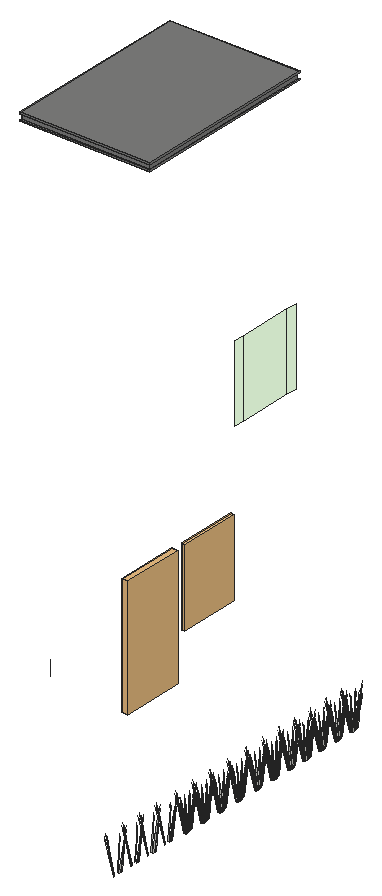
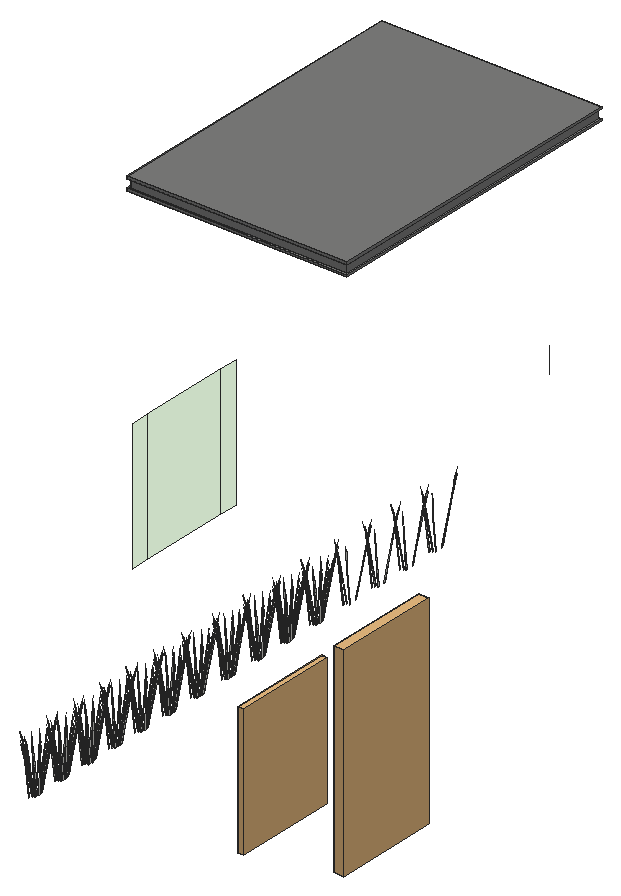
# SketchUp Ruby script. Lengths in inches.
U = 1.inch
M = Sketchup.active_model
def pt(a) = Geom::Point3d.new(a.map { |v| v * U })
def face(e, loops, mat)
  f = e.add_face(loops[0].map { |a| pt(a) })
  loops[1..].each { |l| e.add_face(l.map { |a| pt(a) }).erase! }
  f.material = f.back_material = mat if mat
  f
end
# faces: each face lists its corners as indices into pts; further lists are holes
def faces(e, pts, list, mat = nil) = list.each { |f| face(e, (f[0].is_a?(Array) ? f : [f]).map { |l| l.map { |i| pts[i] } }, mat) }
# xy, xz, yz: faces in a plane at the given z, y or x. An outline is a flat list of corners, or four numbers for a rectangle; further outlines are holes
def ring(l) = l.size == 4 ? [[l[0], l[1]], [l[2], l[1]], [l[2], l[3]], [l[0], l[3]]] : l.each_slice(2).to_a
def flat(e, list, mat, &to3) = list.each { |f| face(e, (f[0].is_a?(Array) ? f : [f]).map { |l| ring(l).map { |u, v| to3.(u, v) } }, mat) }
def xy(e, z, list, mat = nil) = flat(e, list, mat) { |x, y| [x, y, z] }
def xz(e, y, list, mat = nil) = flat(e, list, mat) { |x, z| [x, y, z] }
def yz(e, x, list, mat = nil) = flat(e, list, mat) { |y, z| [x, y, z] }
def lines(e, pts, list) = list.each { |a, b| e.add_line(pt(pts[a]), pt(pts[b])) }
# prism: a flat outline (further loops are holes) pulled along v
def prism(e, loops, v, mat = nil)
  f = face(e, loops, mat); d = Geom::Vector3d.new(v.map { |x| x * U })
  f.pushpull(f.normal.samedirection?(d) ? d.length : -d.length)
end
def box(e, o, s, mat = nil) = prism(e, [[o, [o[0] + s[0], o[1], o[2]], [o[0] + s[0], o[1] + s[1], o[2]], [o[0], o[1] + s[1], o[2]]]], [0, 0, s[2]], mat)
def at(x, y, z, deg = 0) = Geom::Transformation.translation(pt([x, y, z])) * Geom::Transformation.rotation(ORIGIN, Z_AXIS, deg.degrees)
def axes(o, x, y, z) = Geom::Transformation.new([*x, 0, *y, 0, *z, 0, *pt(o).to_a, 1])
def part(name) = M.definitions.add(name)
# library, detail: a bought-in or finely detailed component or shape, given as its bounding box
def library(name, o, s) = part(name).tap { |d| box(d.entities, o, s) }
def detail(e, o, s) = box(e.add_group.entities, o, s)
def put(e, d, t, mat = nil) = e.add_instance(d, t).tap { |i| i.material = mat if mat }
def group(e, t, mat = nil) = e.add_group.tap { |g| g.transformation = t; g.material = mat if mat }.entities
root = M.entities
M.materials.add("Glass_Basic_01").color = [81, 188, 38]
M.materials["Glass_Basic_01"].alpha = 0.25
M.materials.add("LightPink_Translucent").color = [144, 107, 117]
M.materials["LightPink_Translucent"].alpha = 0.75
M.materials.add("ThomThom - Waistcoat2").color = [127, 127, 126]
c1 = part("blade")
p = [[2.15,0.21,22],[0,0.17,0],[0.09,0.45,0],[2.18,0.31,22],[2.29,0.31,22],[0.38,0.45,0],
  [2.48,0.24,33],[2.49,0.24,33],[2.48,0.22,33]]
faces(c1.entities,p,[[0,1,2,3],[4,5,2,3],[6,3,4,7],[8,0,3,6]])
c2 = part("seeds")
p = [[0.3,-0.1,1.38],[-0.01,-0.03,1.59],[-0.01,-0.03,0.03],[0.14,-0.07,-0.07],[0.29,-0.03,3],[0.15,0.01,3.11]]
faces(c2.entities,p,[[0,1,2,3],[1,0,4,5]],"LightPink_Translucent")
c3 = part("blade with seeds")
put(c3.entities,c1,at(0,0,0))
put(c3.entities,c2,axes([2.4,0.25,30.99],[1.5799,-0.05474,1.17369],[-0.12525,1.92788,0.29478],[-0.07173,-0.02425,1.56792]))
c4 = library("porta+4",[0.2,-5.42,1.33],[46.55,4.72,83.21])
c5 = library("mesh-165",[-1596.32,-2661.67,-39.91],[1702.88,1739.15,82.5])
xy(root,354,[[11,219.43,112,365.43]],"ThomThom - Waistcoat2")
xy(root,355,[[12,220.43,111,364.43]])
xy(root,355,[[[11,219.43,112,365.43],[12,220.43,111,364.43]]],"ThomThom - Waistcoat2")
xy(root,359,[[12,220.43,111,364.43]])
xy(root,359,[[11,219.43,111,220.43],[111,219.43,112,365.43],[11,220.43,12,364.43],[11,364.43,111,365.43]],"ThomThom - Waistcoat2")
xy(root,360,[[11,219.43,112,365.43]],"ThomThom - Waistcoat2")
xz(root,219.43,[[11,354,112,355],[11,359,112,360]],"ThomThom - Waistcoat2")
xz(root,220.43,[[12,355,111,359]],"ThomThom - Waistcoat2")
xz(root,364.43,[[12,355,111,359]],"ThomThom - Waistcoat2")
xz(root,365.43,[[11,354,112,355],[11,359,112,360]],"ThomThom - Waistcoat2")
yz(root,11,[[219.43,354,365.43,355],[219.43,359,365.43,360]],"ThomThom - Waistcoat2")
yz(root,12,[[220.43,355,364.43,359]],"ThomThom - Waistcoat2")
yz(root,111,[[220.43,355,364.43,359]],"ThomThom - Waistcoat2")
yz(root,112,[[219.43,354,365.43,355],[219.43,359,365.43,360]],"ThomThom - Waistcoat2")
yz(root,144,[[262.43,168,271.43,228],[271.43,168,313.43,228],[313.43,168,322.43,228]],"Glass_Basic_01")
p = [[183,34.43,108],[183,34.43,120]]
lines(root,p,[[0,1]])
put(root,c3,axes([250.88,80.0625,2.86],[0.14563,0.38283,0.25703],[-0.16629,0.3624,-0.33183],[-0.08449,-0.05514,0.63492]))
put(root,c3,axes([250.97,83.33,2.86],[0.17318,-0.32193,0.25703],[0.16394,0.36759,-0.33183],[-0.02494,0.18677,0.63492]))
put(root,c3,axes([250.67,82.33,2.86],[0.2228,-0.08739,0.25703],[0.05883,0.49954,-0.33183],[-0.06385,0.13418,0.63492]))
put(root,c3,axes([252,83.78,2.86],[-0.03953,-0.49251,0.25703],[0.22598,-0.13005,-0.33183],[0.0607,0.14114,0.63492]))
put(root,c3,axes([252.65,80.84,2.86],[-0.2228,0.08739,0.25703],[-0.05883,-0.49954,-0.33183],[0.06385,-0.13418,0.63492]))
put(root,c3,axes([250.64,81.14,2.86],[0.21272,0.17057,0.25703],[-0.06204,0.49764,-0.33183],[-0.08564,0.04563,0.63492]))
put(root,c3,axes([252.35,79.85,2.86],[-0.17318,0.32193,0.25703],[-0.16394,-0.36759,-0.33183],[0.02494,-0.18677,0.63492]))
put(root,c3,axes([251.33,79.4,2.86],[0.03953,0.49251,0.25703],[-0.22598,0.13005,-0.33183],[-0.0607,-0.14114,0.63492]))
put(root,c3,axes([251.46,100.43,2.86],[0.07716,-0.47021,0.25703],[0.22512,0.13715,-0.33183],[0.02064,0.18932,0.63492]))
put(root,c3,axes([251.87,95.9,2.86],[-0.07716,0.47021,0.25703],[-0.22512,-0.13715,-0.33183],[-0.02064,-0.18932,0.63492]))
put(root,c3,axes([252.45,99.6875,2.86],[-0.14563,-0.38283,0.25703],[0.16629,-0.3624,-0.33183],[0.08449,0.05514,0.63492]))
put(root,c3,axes([252.69,98.62,2.86],[-0.21272,-0.17057,0.25703],[0.06204,-0.49764,-0.33183],[0.08564,-0.04563,0.63492]))
put(root,c3,axes([250.88,96.64,2.86],[0.14563,0.38283,0.25703],[-0.16629,0.3624,-0.33183],[-0.08449,-0.05514,0.63492]))
put(root,c3,axes([250.97,99.9,2.86],[0.17318,-0.32193,0.25703],[0.16394,0.36759,-0.33183],[-0.02494,0.18677,0.63492]))
put(root,c3,axes([250.67,98.91,2.86],[0.2228,-0.08739,0.25703],[0.05883,0.49954,-0.33183],[-0.06385,0.13418,0.63492]))
put(root,c3,axes([252,100.35,2.86],[-0.03953,-0.49251,0.25703],[0.22598,-0.13005,-0.33183],[0.0607,0.14114,0.63492]))
put(root,c3,axes([252.65,97.42,2.86],[-0.2228,0.08739,0.25703],[-0.05883,-0.49954,-0.33183],[0.06385,-0.13418,0.63492]))
put(root,c3,axes([250.64,97.71,2.86],[0.21272,0.17057,0.25703],[-0.06204,0.49764,-0.33183],[-0.08564,0.04563,0.63492]))
put(root,c3,axes([252.35,96.43,2.86],[-0.17318,0.32193,0.25703],[-0.16394,-0.36759,-0.33183],[0.02494,-0.18677,0.63492]))
put(root,c3,axes([251.33,95.97,2.86],[0.03953,0.49251,0.25703],[-0.22598,0.13005,-0.33183],[-0.0607,-0.14114,0.63492]))
put(root,c3,axes([251.46,117.1875,2.86],[0.07716,-0.47021,0.25703],[0.22512,0.13715,-0.33183],[0.02064,0.18932,0.63492]))
put(root,c3,axes([251.87,112.65,2.86],[-0.07716,0.47021,0.25703],[-0.22512,-0.13715,-0.33183],[-0.02064,-0.18932,0.63492]))
put(root,c3,axes([252.45,116.44,2.86],[-0.14563,-0.38283,0.25703],[0.16629,-0.3624,-0.33183],[0.08449,0.05514,0.63492]))
put(root,c3,axes([252.69,115.37,2.86],[-0.21272,-0.17057,0.25703],[0.06204,-0.49764,-0.33183],[0.08564,-0.04563,0.63492]))
put(root,c3,axes([250.88,113.39,2.86],[0.14563,0.38283,0.25703],[-0.16629,0.3624,-0.33183],[-0.08449,-0.05514,0.63492]))
put(root,c3,axes([250.97,116.66,2.86],[0.17318,-0.32193,0.25703],[0.16394,0.36759,-0.33183],[-0.02494,0.18677,0.63492]))
put(root,c3,axes([250.67,115.66,2.86],[0.2228,-0.08739,0.25703],[0.05883,0.49954,-0.33183],[-0.06385,0.13418,0.63492]))
put(root,c3,axes([252,117.11,2.86],[-0.03953,-0.49251,0.25703],[0.22598,-0.13005,-0.33183],[0.0607,0.14114,0.63492]))
put(root,c3,axes([252.65,114.18,2.86],[-0.2228,0.08739,0.25703],[-0.05883,-0.49954,-0.33183],[0.06385,-0.13418,0.63492]))
put(root,c3,axes([250.64,114.47,2.86],[0.21272,0.17057,0.25703],[-0.06204,0.49764,-0.33183],[-0.08564,0.04563,0.63492]))
put(root,c3,axes([252.35,113.18,2.86],[-0.17318,0.32193,0.25703],[-0.16394,-0.36759,-0.33183],[0.02494,-0.18677,0.63492]))
put(root,c3,axes([251.33,112.73,2.86],[0.03953,0.49251,0.25703],[-0.22598,0.13005,-0.33183],[-0.0607,-0.14114,0.63492]))
put(root,c3,axes([251.46,134.63,2.86],[0.07716,-0.47021,0.25703],[0.22512,0.13715,-0.33183],[0.02064,0.18932,0.63492]))
put(root,c3,axes([251.87,130.1,2.86],[-0.07716,0.47021,0.25703],[-0.22512,-0.13715,-0.33183],[-0.02064,-0.18932,0.63492]))
put(root,c3,axes([252.45,133.89,2.86],[-0.14563,-0.38283,0.25703],[0.16629,-0.3624,-0.33183],[0.08449,0.05514,0.63492]))
put(root,c3,axes([252.69,132.82,2.86],[-0.21272,-0.17057,0.25703],[0.06204,-0.49764,-0.33183],[0.08564,-0.04563,0.63492]))
put(root,c3,axes([250.88,130.84,2.86],[0.14563,0.38283,0.25703],[-0.16629,0.3624,-0.33183],[-0.08449,-0.05514,0.63492]))
put(root,c3,axes([250.97,134.1,2.86],[0.17318,-0.32193,0.25703],[0.16394,0.36759,-0.33183],[-0.02494,0.18677,0.63492]))
put(root,c3,axes([250.67,133.11,2.86],[0.2228,-0.08739,0.25703],[0.05883,0.49954,-0.33183],[-0.06385,0.13418,0.63492]))
put(root,c3,axes([252,134.55,2.86],[-0.03953,-0.49251,0.25703],[0.22598,-0.13005,-0.33183],[0.0607,0.14114,0.63492]))
put(root,c3,axes([252.65,131.62,2.86],[-0.2228,0.08739,0.25703],[-0.05883,-0.49954,-0.33183],[0.06385,-0.13418,0.63492]))
put(root,c3,axes([250.64,131.91,2.86],[0.21272,0.17057,0.25703],[-0.06204,0.49764,-0.33183],[-0.08564,0.04563,0.63492]))
put(root,c3,axes([252.35,130.625,2.86],[-0.17318,0.32193,0.25703],[-0.16394,-0.36759,-0.33183],[0.02494,-0.18677,0.63492]))
put(root,c3,axes([251.33,130.18,2.86],[0.03953,0.49251,0.25703],[-0.22598,0.13005,-0.33183],[-0.0607,-0.14114,0.63492]))
put(root,c3,axes([251.46,152.28,2.86],[0.07716,-0.47021,0.25703],[0.22512,0.13715,-0.33183],[0.02064,0.18932,0.63492]))
put(root,c3,axes([251.87,147.74,2.86],[-0.07716,0.47021,0.25703],[-0.22512,-0.13715,-0.33183],[-0.02064,-0.18932,0.63492]))
put(root,c3,axes([252.45,151.53,2.86],[-0.14563,-0.38283,0.25703],[0.16629,-0.3624,-0.33183],[0.08449,0.05514,0.63492]))
put(root,c3,axes([252.69,150.46,2.86],[-0.21272,-0.17057,0.25703],[0.06204,-0.49764,-0.33183],[0.08564,-0.04563,0.63492]))
put(root,c3,axes([250.88,148.48,2.86],[0.14563,0.38283,0.25703],[-0.16629,0.3624,-0.33183],[-0.08449,-0.05514,0.63492]))
put(root,c3,axes([250.97,151.75,2.86],[0.17318,-0.32193,0.25703],[0.16394,0.36759,-0.33183],[-0.02494,0.18677,0.63492]))
put(root,c3,axes([250.67,150.75,2.86],[0.2228,-0.08739,0.25703],[0.05883,0.49954,-0.33183],[-0.06385,0.13418,0.63492]))
put(root,c3,axes([252,152.2,2.86],[-0.03953,-0.49251,0.25703],[0.22598,-0.13005,-0.33183],[0.0607,0.14114,0.63492]))
put(root,c3,axes([252.65,149.26,2.86],[-0.2228,0.08739,0.25703],[-0.05883,-0.49954,-0.33183],[0.06385,-0.13418,0.63492]))
put(root,c3,axes([250.64,149.56,2.86],[0.21272,0.17057,0.25703],[-0.06204,0.49764,-0.33183],[-0.08564,0.04563,0.63492]))
put(root,c3,axes([252.35,148.27,2.86],[-0.17318,0.32193,0.25703],[-0.16394,-0.36759,-0.33183],[0.02494,-0.18677,0.63492]))
put(root,c3,axes([251.33,147.82,2.86],[0.03953,0.49251,0.25703],[-0.22598,0.13005,-0.33183],[-0.0607,-0.14114,0.63492]))
put(root,c3,axes([251.46,168.55,2.86],[0.07716,-0.47021,0.25703],[0.22512,0.13715,-0.33183],[0.02064,0.18932,0.63492]))
put(root,c3,axes([251.87,164.01,2.86],[-0.07716,0.47021,0.25703],[-0.22512,-0.13715,-0.33183],[-0.02064,-0.18932,0.63492]))
put(root,c3,axes([252.45,167.8,2.86],[-0.14563,-0.38283,0.25703],[0.16629,-0.3624,-0.33183],[0.08449,0.05514,0.63492]))
put(root,c3,axes([252.69,166.73,2.86],[-0.21272,-0.17057,0.25703],[0.06204,-0.49764,-0.33183],[0.08564,-0.04563,0.63492]))
put(root,c3,axes([250.88,164.75,2.86],[0.14563,0.38283,0.25703],[-0.16629,0.3624,-0.33183],[-0.08449,-0.05514,0.63492]))
put(root,c3,axes([250.97,168.02,2.86],[0.17318,-0.32193,0.25703],[0.16394,0.36759,-0.33183],[-0.02494,0.18677,0.63492]))
put(root,c3,axes([250.67,167.02,2.86],[0.2228,-0.08739,0.25703],[0.05883,0.49954,-0.33183],[-0.06385,0.13418,0.63492]))
put(root,c3,axes([252,168.47,2.86],[-0.03953,-0.49251,0.25703],[0.22598,-0.13005,-0.33183],[0.0607,0.14114,0.63492]))
put(root,c3,axes([252.65,165.53,2.86],[-0.2228,0.08739,0.25703],[-0.05883,-0.49954,-0.33183],[0.06385,-0.13418,0.63492]))
put(root,c3,axes([250.64,165.83,2.86],[0.21272,0.17057,0.25703],[-0.06204,0.49764,-0.33183],[-0.08564,0.04563,0.63492]))
put(root,c3,axes([252.35,164.54,2.86],[-0.17318,0.32193,0.25703],[-0.16394,-0.36759,-0.33183],[0.02494,-0.18677,0.63492]))
put(root,c3,axes([251.33,164.09,2.86],[0.03953,0.49251,0.25703],[-0.22598,0.13005,-0.33183],[-0.0607,-0.14114,0.63492]))
put(root,c3,axes([251.46,184.4,2.86],[0.07716,-0.47021,0.25703],[0.22512,0.13715,-0.33183],[0.02064,0.18932,0.63492]))
put(root,c3,axes([251.87,179.86,2.86],[-0.07716,0.47021,0.25703],[-0.22512,-0.13715,-0.33183],[-0.02064,-0.18932,0.63492]))
put(root,c3,axes([252.45,183.65,2.86],[-0.14563,-0.38283,0.25703],[0.16629,-0.3624,-0.33183],[0.08449,0.05514,0.63492]))
put(root,c3,axes([252.69,182.58,2.86],[-0.21272,-0.17057,0.25703],[0.06204,-0.49764,-0.33183],[0.08564,-0.04563,0.63492]))
put(root,c3,axes([250.88,180.6,2.86],[0.14563,0.38283,0.25703],[-0.16629,0.3624,-0.33183],[-0.08449,-0.05514,0.63492]))
put(root,c3,axes([250.97,183.87,2.86],[0.17318,-0.32193,0.25703],[0.16394,0.36759,-0.33183],[-0.02494,0.18677,0.63492]))
put(root,c3,axes([250.67,182.87,2.86],[0.2228,-0.08739,0.25703],[0.05883,0.49954,-0.33183],[-0.06385,0.13418,0.63492]))
put(root,c3,axes([252,184.32,2.86],[-0.03953,-0.49251,0.25703],[0.22598,-0.13005,-0.33183],[0.0607,0.14114,0.63492]))
put(root,c3,axes([252.65,181.39,2.86],[-0.2228,0.08739,0.25703],[-0.05883,-0.49954,-0.33183],[0.06385,-0.13418,0.63492]))
put(root,c3,axes([250.64,181.68,2.86],[0.21272,0.17057,0.25703],[-0.06204,0.49764,-0.33183],[-0.08564,0.04563,0.63492]))
put(root,c3,axes([252.35,180.39,2.86],[-0.17318,0.32193,0.25703],[-0.16394,-0.36759,-0.33183],[0.02494,-0.18677,0.63492]))
put(root,c3,axes([251.33,179.9375,2.86],[0.03953,0.49251,0.25703],[-0.22598,0.13005,-0.33183],[-0.0607,-0.14114,0.63492]))
put(root,c3,axes([251.46,199.38,2.86],[0.07716,-0.47021,0.25703],[0.22512,0.13715,-0.33183],[0.02064,0.18932,0.63492]))
put(root,c3,axes([251.87,194.85,2.86],[-0.07716,0.47021,0.25703],[-0.22512,-0.13715,-0.33183],[-0.02064,-0.18932,0.63492]))
put(root,c3,axes([252.45,198.64,2.86],[-0.14563,-0.38283,0.25703],[0.16629,-0.3624,-0.33183],[0.08449,0.05514,0.63492]))
put(root,c3,axes([252.69,197.57,2.86],[-0.21272,-0.17057,0.25703],[0.06204,-0.49764,-0.33183],[0.08564,-0.04563,0.63492]))
put(root,c3,axes([250.88,195.59,2.86],[0.14563,0.38283,0.25703],[-0.16629,0.3624,-0.33183],[-0.08449,-0.05514,0.63492]))
put(root,c3,axes([250.97,198.85,2.86],[0.17318,-0.32193,0.25703],[0.16394,0.36759,-0.33183],[-0.02494,0.18677,0.63492]))
put(root,c3,axes([250.67,197.86,2.86],[0.2228,-0.08739,0.25703],[0.05883,0.49954,-0.33183],[-0.06385,0.13418,0.63492]))
put(root,c3,axes([252,199.3,2.86],[-0.03953,-0.49251,0.25703],[0.22598,-0.13005,-0.33183],[0.0607,0.14114,0.63492]))
put(root,c3,axes([252.65,196.37,2.86],[-0.2228,0.08739,0.25703],[-0.05883,-0.49954,-0.33183],[0.06385,-0.13418,0.63492]))
put(root,c3,axes([250.64,196.66,2.86],[0.21272,0.17057,0.25703],[-0.06204,0.49764,-0.33183],[-0.08564,0.04563,0.63492]))
put(root,c3,axes([252.35,195.375,2.86],[-0.17318,0.32193,0.25703],[-0.16394,-0.36759,-0.33183],[0.02494,-0.18677,0.63492]))
put(root,c3,axes([251.33,194.93,2.86],[0.03953,0.49251,0.25703],[-0.22598,0.13005,-0.33183],[-0.0607,-0.14114,0.63492]))
put(root,c3,axes([251.46,214.64,2.86],[0.07716,-0.47021,0.25703],[0.22512,0.13715,-0.33183],[0.02064,0.18932,0.63492]))
put(root,c3,axes([251.87,210.1,2.86],[-0.07716,0.47021,0.25703],[-0.22512,-0.13715,-0.33183],[-0.02064,-0.18932,0.63492]))
put(root,c3,axes([252.45,213.89,2.86],[-0.14563,-0.38283,0.25703],[0.16629,-0.3624,-0.33183],[0.08449,0.05514,0.63492]))
put(root,c3,axes([252.69,212.82,2.86],[-0.21272,-0.17057,0.25703],[0.06204,-0.49764,-0.33183],[0.08564,-0.04563,0.63492]))
put(root,c3,axes([250.88,210.84,2.86],[0.14563,0.38283,0.25703],[-0.16629,0.3624,-0.33183],[-0.08449,-0.05514,0.63492]))
put(root,c3,axes([250.97,214.11,2.86],[0.17318,-0.32193,0.25703],[0.16394,0.36759,-0.33183],[-0.02494,0.18677,0.63492]))
put(root,c3,axes([250.67,213.11,2.86],[0.2228,-0.08739,0.25703],[0.05883,0.49954,-0.33183],[-0.06385,0.13418,0.63492]))
put(root,c3,axes([252,214.56,2.86],[-0.03953,-0.49251,0.25703],[0.22598,-0.13005,-0.33183],[0.0607,0.14114,0.63492]))
put(root,c3,axes([252.65,211.625,2.86],[-0.2228,0.08739,0.25703],[-0.05883,-0.49954,-0.33183],[0.06385,-0.13418,0.63492]))
put(root,c3,axes([250.64,211.92,2.86],[0.21272,0.17057,0.25703],[-0.06204,0.49764,-0.33183],[-0.08564,0.04563,0.63492]))
put(root,c3,axes([252.35,210.63,2.86],[-0.17318,0.32193,0.25703],[-0.16394,-0.36759,-0.33183],[0.02494,-0.18677,0.63492]))
put(root,c3,axes([251.33,210.18,2.86],[0.03953,0.49251,0.25703],[-0.22598,0.13005,-0.33183],[-0.0607,-0.14114,0.63492]))
put(root,c3,axes([251.46,230.15,2.86],[0.07716,-0.47021,0.25703],[0.22512,0.13715,-0.33183],[0.02064,0.18932,0.63492]))
put(root,c3,axes([251.87,225.61,2.86],[-0.07716,0.47021,0.25703],[-0.22512,-0.13715,-0.33183],[-0.02064,-0.18932,0.63492]))
put(root,c3,axes([252.45,229.4,2.86],[-0.14563,-0.38283,0.25703],[0.16629,-0.3624,-0.33183],[0.08449,0.05514,0.63492]))
put(root,c3,axes([252.69,228.33,2.86],[-0.21272,-0.17057,0.25703],[0.06204,-0.49764,-0.33183],[0.08564,-0.04563,0.63492]))
put(root,c3,axes([250.88,226.35,2.86],[0.14563,0.38283,0.25703],[-0.16629,0.3624,-0.33183],[-0.08449,-0.05514,0.63492]))
put(root,c3,axes([250.97,229.62,2.86],[0.17318,-0.32193,0.25703],[0.16394,0.36759,-0.33183],[-0.02494,0.18677,0.63492]))
put(root,c3,axes([250.67,228.62,2.86],[0.2228,-0.08739,0.25703],[0.05883,0.49954,-0.33183],[-0.06385,0.13418,0.63492]))
put(root,c3,axes([252,230.07,2.86],[-0.03953,-0.49251,0.25703],[0.22598,-0.13005,-0.33183],[0.0607,0.14114,0.63492]))
put(root,c3,axes([252.65,227.13,2.86],[-0.2228,0.08739,0.25703],[-0.05883,-0.49954,-0.33183],[0.06385,-0.13418,0.63492]))
put(root,c3,axes([250.64,227.43,2.86],[0.21272,0.17057,0.25703],[-0.06204,0.49764,-0.33183],[-0.08564,0.04563,0.63492]))
put(root,c3,axes([252.35,226.14,2.86],[-0.17318,0.32193,0.25703],[-0.16394,-0.36759,-0.33183],[0.02494,-0.18677,0.63492]))
put(root,c3,axes([251.33,225.6875,2.86],[0.03953,0.49251,0.25703],[-0.22598,0.13005,-0.33183],[-0.0607,-0.14114,0.63492]))
put(root,c3,axes([251.46,245.23,2.86],[0.07716,-0.47021,0.25703],[0.22512,0.13715,-0.33183],[0.02064,0.18932,0.63492]))
put(root,c3,axes([251.87,240.69,2.86],[-0.07716,0.47021,0.25703],[-0.22512,-0.13715,-0.33183],[-0.02064,-0.18932,0.63492]))
put(root,c3,axes([252.45,244.49,2.86],[-0.14563,-0.38283,0.25703],[0.16629,-0.3624,-0.33183],[0.08449,0.05514,0.63492]))
put(root,c3,axes([252.69,243.41,2.86],[-0.21272,-0.17057,0.25703],[0.06204,-0.49764,-0.33183],[0.08564,-0.04563,0.63492]))
put(root,c3,axes([250.88,241.4375,2.86],[0.14563,0.38283,0.25703],[-0.16629,0.3624,-0.33183],[-0.08449,-0.05514,0.63492]))
put(root,c3,axes([250.97,244.7,2.86],[0.17318,-0.32193,0.25703],[0.16394,0.36759,-0.33183],[-0.02494,0.18677,0.63492]))
put(root,c3,axes([250.67,243.7,2.86],[0.2228,-0.08739,0.25703],[0.05883,0.49954,-0.33183],[-0.06385,0.13418,0.63492]))
put(root,c3,axes([252,245.15,2.86],[-0.03953,-0.49251,0.25703],[0.22598,-0.13005,-0.33183],[0.0607,0.14114,0.63492]))
put(root,c3,axes([252.65,242.22,2.86],[-0.2228,0.08739,0.25703],[-0.05883,-0.49954,-0.33183],[0.06385,-0.13418,0.63492]))
put(root,c3,axes([250.64,242.51,2.86],[0.21272,0.17057,0.25703],[-0.06204,0.49764,-0.33183],[-0.08564,0.04563,0.63492]))
put(root,c3,axes([252.35,241.22,2.86],[-0.17318,0.32193,0.25703],[-0.16394,-0.36759,-0.33183],[0.02494,-0.18677,0.63492]))
put(root,c3,axes([251.33,240.77,2.86],[0.03953,0.49251,0.25703],[-0.22598,0.13005,-0.33183],[-0.0607,-0.14114,0.63492]))
put(root,c3,axes([251.46,15.75,2.87],[-0.25221,-0.15985,0.38672],[0.08624,-0.52553,0.31887],[0.01516,0.20667,0.80022]))
put(root,c3,axes([251.46,32.61,2.87],[-0.25221,-0.15985,0.38672],[0.08624,-0.52553,0.31887],[0.01516,0.20667,0.80022]))
put(root,c3,axes([251.46,48.77,2.87],[-0.25221,-0.15985,0.38672],[0.08624,-0.52553,0.31887],[0.01516,0.20667,0.80022]))
put(root,c3,axes([251.46,65.22,2.87],[-0.25221,-0.15985,0.38672],[0.08624,-0.52553,0.31887],[0.01516,0.20667,0.80022]))
put(root,c3,axes([251.46,84.24,2.87],[-0.25221,-0.15985,0.38672],[0.08624,-0.52553,0.31887],[0.01516,0.20667,0.80022]))
put(root,c3,axes([251.46,100.82,2.87],[-0.25221,-0.15985,0.38672],[0.08624,-0.52553,0.31887],[0.01516,0.20667,0.80022]))
put(root,c3,axes([251.46,117.57,2.87],[-0.25221,-0.15985,0.38672],[0.08624,-0.52553,0.31887],[0.01516,0.20667,0.80022]))
put(root,c3,axes([251.46,135.02,2.87],[-0.25221,-0.15985,0.38672],[0.08624,-0.52553,0.31887],[0.01516,0.20667,0.80022]))
put(root,c3,axes([251.46,152.66,2.87],[-0.25221,-0.15985,0.38672],[0.08624,-0.52553,0.31887],[0.01516,0.20667,0.80022]))
put(root,c3,axes([251.46,168.93,2.87],[-0.25221,-0.15985,0.38672],[0.08624,-0.52553,0.31887],[0.01516,0.20667,0.80022]))
put(root,c3,axes([251.46,184.78,2.87],[-0.25221,-0.15985,0.38672],[0.08624,-0.52553,0.31887],[0.01516,0.20667,0.80022]))
put(root,c3,axes([251.46,199.77,2.87],[-0.25221,-0.15985,0.38672],[0.08624,-0.52553,0.31887],[0.01516,0.20667,0.80022]))
put(root,c3,axes([251.46,215.02,2.87],[-0.25221,-0.15985,0.38672],[0.08624,-0.52553,0.31887],[0.01516,0.20667,0.80022]))
put(root,c3,axes([251.46,230.53,2.87],[-0.25221,-0.15985,0.38672],[0.08624,-0.52553,0.31887],[0.01516,0.20667,0.80022]))
put(root,c3,axes([251.46,245.62,2.87],[-0.25221,-0.15985,0.38672],[0.08624,-0.52553,0.31887],[0.01516,0.20667,0.80022]))
put(root,c3,axes([250.65,11.22,2.89],[0.21138,-0.45125,0.3902],[0.1823,0.47921,0.32174],[-0.09917,-0.08324,0.80743]))
put(root,c3,axes([251.23,10.32,2.89],[0.28513,-0.15716,0.3902],[0.04948,0.6165,0.32174],[-0.06706,-0.1817,0.80743]))
put(root,c3,axes([250.65,28.09,2.89],[0.21138,-0.45125,0.3902],[0.1823,0.47921,0.32174],[-0.09917,-0.08324,0.80743]))
put(root,c3,axes([251.23,27.19,2.89],[0.28513,-0.15716,0.3902],[0.04948,0.6165,0.32174],[-0.06706,-0.1817,0.80743]))
put(root,c3,axes([250.65,44.24,2.89],[0.21138,-0.45125,0.3902],[0.1823,0.47921,0.32174],[-0.09917,-0.08324,0.80743]))
put(root,c3,axes([251.23,43.34,2.89],[0.28513,-0.15716,0.3902],[0.04948,0.6165,0.32174],[-0.06706,-0.1817,0.80743]))
put(root,c3,axes([250.65,60.69,2.89],[0.21138,-0.45125,0.3902],[0.1823,0.47921,0.32174],[-0.09917,-0.08324,0.80743]))
put(root,c3,axes([251.23,59.79,2.89],[0.28513,-0.15716,0.3902],[0.04948,0.6165,0.32174],[-0.06706,-0.1817,0.80743]))
put(root,c3,axes([250.65,79.72,2.89],[0.21138,-0.45125,0.3902],[0.1823,0.47921,0.32174],[-0.09917,-0.08324,0.80743]))
put(root,c3,axes([251.23,78.82,2.89],[0.28513,-0.15716,0.3902],[0.04948,0.6165,0.32174],[-0.06706,-0.1817,0.80743]))
put(root,c3,axes([250.65,96.3,2.89],[0.21138,-0.45125,0.3902],[0.1823,0.47921,0.32174],[-0.09917,-0.08324,0.80743]))
put(root,c3,axes([251.23,95.39,2.89],[0.28513,-0.15716,0.3902],[0.04948,0.6165,0.32174],[-0.06706,-0.1817,0.80743]))
put(root,c3,axes([250.65,113.05,2.89],[0.21138,-0.45125,0.3902],[0.1823,0.47921,0.32174],[-0.09917,-0.08324,0.80743]))
put(root,c3,axes([251.23,112.15,2.89],[0.28513,-0.15716,0.3902],[0.04948,0.6165,0.32174],[-0.06706,-0.1817,0.80743]))
put(root,c3,axes([250.65,130.5,2.89],[0.21138,-0.45125,0.3902],[0.1823,0.47921,0.32174],[-0.09917,-0.08324,0.80743]))
put(root,c3,axes([251.23,129.6,2.89],[0.28513,-0.15716,0.3902],[0.04948,0.6165,0.32174],[-0.06706,-0.1817,0.80743]))
put(root,c3,axes([250.65,148.14,2.89],[0.21138,-0.45125,0.3902],[0.1823,0.47921,0.32174],[-0.09917,-0.08324,0.80743]))
put(root,c3,axes([251.23,147.24,2.89],[0.28513,-0.15716,0.3902],[0.04948,0.6165,0.32174],[-0.06706,-0.1817,0.80743]))
put(root,c3,axes([250.65,164.41,2.89],[0.21138,-0.45125,0.3902],[0.1823,0.47921,0.32174],[-0.09917,-0.08324,0.80743]))
put(root,c3,axes([251.23,163.51,2.89],[0.28513,-0.15716,0.3902],[0.04948,0.6165,0.32174],[-0.06706,-0.1817,0.80743]))
put(root,c3,axes([250.65,180.26,2.89],[0.21138,-0.45125,0.3902],[0.1823,0.47921,0.32174],[-0.09917,-0.08324,0.80743]))
put(root,c3,axes([251.23,179.36,2.89],[0.28513,-0.15716,0.3902],[0.04948,0.6165,0.32174],[-0.06706,-0.1817,0.80743]))
put(root,c3,axes([250.65,195.25,2.89],[0.21138,-0.45125,0.3902],[0.1823,0.47921,0.32174],[-0.09917,-0.08324,0.80743]))
put(root,c3,axes([251.23,194.35,2.89],[0.28513,-0.15716,0.3902],[0.04948,0.6165,0.32174],[-0.06706,-0.1817,0.80743]))
put(root,c3,axes([250.65,210.5,2.89],[0.21138,-0.45125,0.3902],[0.1823,0.47921,0.32174],[-0.09917,-0.08324,0.80743]))
put(root,c3,axes([251.23,209.6,2.89],[0.28513,-0.15716,0.3902],[0.04948,0.6165,0.32174],[-0.06706,-0.1817,0.80743]))
put(root,c3,axes([250.65,226.01,2.89],[0.21138,-0.45125,0.3902],[0.1823,0.47921,0.32174],[-0.09917,-0.08324,0.80743]))
put(root,c3,axes([251.23,225.11,2.89],[0.28513,-0.15716,0.3902],[0.04948,0.6165,0.32174],[-0.06706,-0.1817,0.80743]))
put(root,c3,axes([250.65,241.09,2.89],[0.21138,-0.45125,0.3902],[0.1823,0.47921,0.32174],[-0.09917,-0.08324,0.80743]))
put(root,c3,axes([251.23,240.19,2.89],[0.28513,-0.15716,0.3902],[0.04948,0.6165,0.32174],[-0.06706,-0.1817,0.80743]))
put(root,c4,axes([127.16,172.22,1.47],[0,1.05,0],[-1,0,0],[0,0,1.12]))
put(root,c3,axes([251.76,17.04,3.29],[0.17688,-0.35078,-0.04709],[0.16207,0.38418,-0.21349],[0.01141,0.10886,0.70419]))
put(root,c3,axes([250.17,15.25,3.29],[0.22586,0.16322,-0.04709],[-0.06948,0.50235,-0.21349],[-0.03694,0.07627,0.70419]))
put(root,c3,axes([251.76,33.91,3.29],[0.17688,-0.35078,-0.04709],[0.16207,0.38418,-0.21349],[0.01141,0.10886,0.70419]))
put(root,c3,axes([250.17,32.12,3.29],[0.22586,0.16322,-0.04709],[-0.06948,0.50235,-0.21349],[-0.03694,0.07627,0.70419]))
put(root,c3,axes([251.76,50.06,3.29],[0.17688,-0.35078,-0.04709],[0.16207,0.38418,-0.21349],[0.01141,0.10886,0.70419]))
put(root,c3,axes([250.17,48.27,3.29],[0.22586,0.16322,-0.04709],[-0.06948,0.50235,-0.21349],[-0.03694,0.07627,0.70419]))
put(root,c3,axes([251.76,66.51,3.29],[0.17688,-0.35078,-0.04709],[0.16207,0.38418,-0.21349],[0.01141,0.10886,0.70419]))
put(root,c3,axes([250.17,64.72,3.29],[0.22586,0.16322,-0.04709],[-0.06948,0.50235,-0.21349],[-0.03694,0.07627,0.70419]))
put(root,c3,axes([251.76,85.53,3.29],[0.17688,-0.35078,-0.04709],[0.16207,0.38418,-0.21349],[0.01141,0.10886,0.70419]))
put(root,c3,axes([250.17,83.75,3.29],[0.22586,0.16322,-0.04709],[-0.06948,0.50235,-0.21349],[-0.03694,0.07627,0.70419]))
put(root,c3,axes([251.76,102.11,3.29],[0.17688,-0.35078,-0.04709],[0.16207,0.38418,-0.21349],[0.01141,0.10886,0.70419]))
put(root,c3,axes([250.17,100.33,3.29],[0.22586,0.16322,-0.04709],[-0.06948,0.50235,-0.21349],[-0.03694,0.07627,0.70419]))
put(root,c3,axes([251.76,118.87,3.29],[0.17688,-0.35078,-0.04709],[0.16207,0.38418,-0.21349],[0.01141,0.10886,0.70419]))
put(root,c3,axes([250.17,117.08,3.29],[0.22586,0.16322,-0.04709],[-0.06948,0.50235,-0.21349],[-0.03694,0.07627,0.70419]))
put(root,c3,axes([251.76,136.31,3.29],[0.17688,-0.35078,-0.04709],[0.16207,0.38418,-0.21349],[0.01141,0.10886,0.70419]))
put(root,c3,axes([250.17,134.53,3.29],[0.22586,0.16322,-0.04709],[-0.06948,0.50235,-0.21349],[-0.03694,0.07627,0.70419]))
put(root,c3,axes([251.76,153.95,3.29],[0.17688,-0.35078,-0.04709],[0.16207,0.38418,-0.21349],[0.01141,0.10886,0.70419]))
put(root,c3,axes([250.17,152.17,3.29],[0.22586,0.16322,-0.04709],[-0.06948,0.50235,-0.21349],[-0.03694,0.07627,0.70419]))
put(root,c3,axes([251.76,170.22,3.29],[0.17688,-0.35078,-0.04709],[0.16207,0.38418,-0.21349],[0.01141,0.10886,0.70419]))
put(root,c3,axes([250.17,168.4375,3.29],[0.22586,0.16322,-0.04709],[-0.06948,0.50235,-0.21349],[-0.03694,0.07627,0.70419]))
put(root,c3,axes([251.76,186.07,3.29],[0.17688,-0.35078,-0.04709],[0.16207,0.38418,-0.21349],[0.01141,0.10886,0.70419]))
put(root,c3,axes([250.17,184.29,3.29],[0.22586,0.16322,-0.04709],[-0.06948,0.50235,-0.21349],[-0.03694,0.07627,0.70419]))
put(root,c3,axes([251.76,201.06,3.29],[0.17688,-0.35078,-0.04709],[0.16207,0.38418,-0.21349],[0.01141,0.10886,0.70419]))
put(root,c3,axes([250.17,199.28,3.29],[0.22586,0.16322,-0.04709],[-0.06948,0.50235,-0.21349],[-0.03694,0.07627,0.70419]))
put(root,c3,axes([251.76,216.3125,3.29],[0.17688,-0.35078,-0.04709],[0.16207,0.38418,-0.21349],[0.01141,0.10886,0.70419]))
put(root,c3,axes([250.17,214.53,3.29],[0.22586,0.16322,-0.04709],[-0.06948,0.50235,-0.21349],[-0.03694,0.07627,0.70419]))
put(root,c3,axes([251.76,231.82,3.29],[0.17688,-0.35078,-0.04709],[0.16207,0.38418,-0.21349],[0.01141,0.10886,0.70419]))
put(root,c3,axes([250.17,230.04,3.29],[0.22586,0.16322,-0.04709],[-0.06948,0.50235,-0.21349],[-0.03694,0.07627,0.70419]))
put(root,c3,axes([251.76,246.91,3.29],[0.17688,-0.35078,-0.04709],[0.16207,0.38418,-0.21349],[0.01141,0.10886,0.70419]))
put(root,c3,axes([250.17,245.125,3.29],[0.22586,0.16322,-0.04709],[-0.06948,0.50235,-0.21349],[-0.03694,0.07627,0.70419]))
g1 = group(root,at(130.1,266.12,98.42))
put(g1,c5,axes([0.11,8.31,29.78],[0,0.02819,0],[0,0,0.03465],[0.03028,0,0]))
